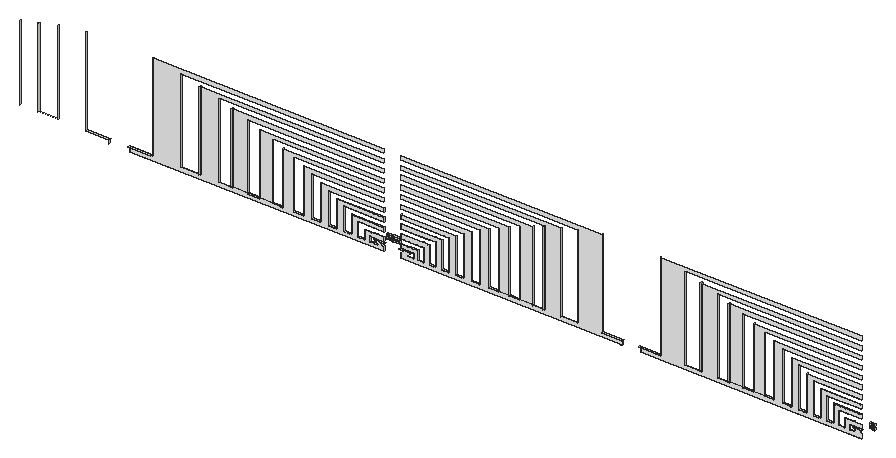
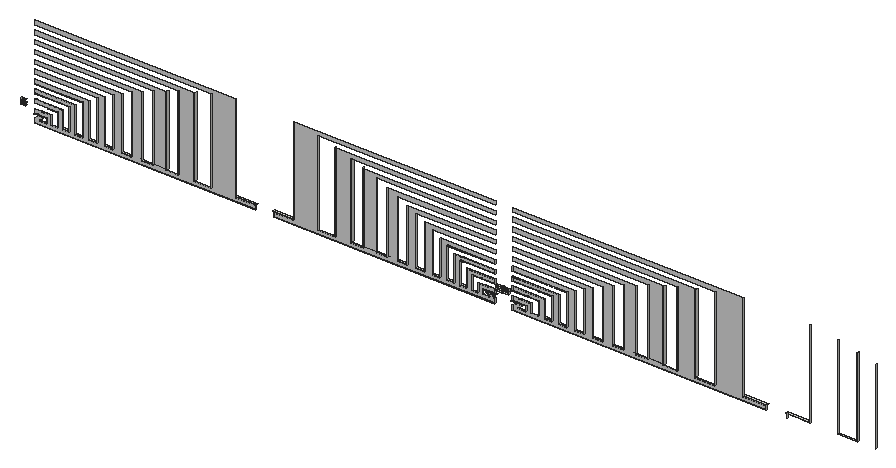
# SketchUp Ruby script. Lengths in inches.
U = 1.inch
M = Sketchup.active_model
def pt(a) = Geom::Point3d.new(a.map { |v| v * U })
def face(e, loops, mat)
  f = e.add_face(loops[0].map { |a| pt(a) })
  loops[1..].each { |l| e.add_face(l.map { |a| pt(a) }).erase! }
  f.material = f.back_material = mat if mat
  f
end
# faces: each face lists its corners as indices into pts; further lists are holes
def faces(e, pts, list, mat = nil) = list.each { |f| face(e, (f[0].is_a?(Array) ? f : [f]).map { |l| l.map { |i| pts[i] } }, mat) }
# xy, xz, yz: faces in a plane at the given z, y or x. An outline is a flat list of corners, or four numbers for a rectangle; further outlines are holes
def ring(l) = l.size == 4 ? [[l[0], l[1]], [l[2], l[1]], [l[2], l[3]], [l[0], l[3]]] : l.each_slice(2).to_a
def flat(e, list, mat, &to3) = list.each { |f| face(e, (f[0].is_a?(Array) ? f : [f]).map { |l| ring(l).map { |u, v| to3.(u, v) } }, mat) }
def xy(e, z, list, mat = nil) = flat(e, list, mat) { |x, y| [x, y, z] }
def xz(e, y, list, mat = nil) = flat(e, list, mat) { |x, z| [x, y, z] }
def yz(e, x, list, mat = nil) = flat(e, list, mat) { |y, z| [x, y, z] }
def lines(e, pts, list) = list.each { |a, b| e.add_line(pt(pts[a]), pt(pts[b])) }
# prism: a flat outline (further loops are holes) pulled along v
def prism(e, loops, v, mat = nil)
  f = face(e, loops, mat); d = Geom::Vector3d.new(v.map { |x| x * U })
  f.pushpull(f.normal.samedirection?(d) ? d.length : -d.length)
end
def box(e, o, s, mat = nil) = prism(e, [[o, [o[0] + s[0], o[1], o[2]], [o[0] + s[0], o[1] + s[1], o[2]], [o[0], o[1] + s[1], o[2]]]], [0, 0, s[2]], mat)
def at(x, y, z, deg = 0) = Geom::Transformation.translation(pt([x, y, z])) * Geom::Transformation.rotation(ORIGIN, Z_AXIS, deg.degrees)
def axes(o, x, y, z) = Geom::Transformation.new([*x, 0, *y, 0, *z, 0, *pt(o).to_a, 1])
def part(name) = M.definitions.add(name)
# library, detail: a bought-in or finely detailed component or shape, given as its bounding box
def library(name, o, s) = part(name).tap { |d| box(d.entities, o, s) }
def detail(e, o, s) = box(e.add_group.entities, o, s)
def put(e, d, t, mat = nil) = e.add_instance(d, t).tap { |i| i.material = mat if mat }
def group(e, t, mat = nil) = e.add_group.tap { |g| g.transformation = t; g.material = mat if mat }.entities
root = M.entities
M.materials.add("[Color_000]").color = [255, 255, 255]
xy(root,0.49,[[835.26,13.81,1012.48,14.31],[1024.39,13.81,1178.58,14.31],[1191.27,13.81,1345.46,14.31]])
xy(root,3.2,[[771.16,13.81,785.19,14.31],[804.64,13.81,816.11,14.31],[816.11,13.81,820.67,14.31],[835.26,13.81,839.82,14.31],[839.82,13.81,851.28,14.31],
  [870.74,13.81,884.76,14.31],[897.07,13.81,907.12,14.31],[917.52,13.81,926.1,14.31],[934.55,13.81,942.21,14.31],[949.3125,13.81,956.23,14.31],
  [962.35,13.81,968.64,14.31],[974.05,13.81,979.79,14.31],[984.5625,13.81,989.91,14.31],[993.96,13.81,999.18,14.31],[1002.58,13.81,1008.33,14.31],
  [1028,13.81,1033,14.31],[1035.96,13.81,1040.51,14.31],[1044.03,13.81,1048.68,14.31],[1052.83,13.81,1057.83,14.31],[1062.53,13.81,1068,14.31],
  [1073.33,13.81,1079.35,14.31],[1085.53,13.81,1092.19,14.31],[1099.55,13.81,1107,14.31],[1116.06,13.81,1124.8,14.31],[1135.51,13.81,1147.71,14.31],
  [1164.63,13.81,1174.61,14.31],[1174.61,13.81,1178.58,14.31],[1191.27,13.81,1195.24,14.31],[1195.24,13.81,1205.21,14.31],[1222.14,13.81,1234.34,14.31],
  [1245.05,13.81,1253.79,14.31],[1262.84,13.81,1270.3,14.31],[1277.65,13.81,1284.32,14.31],[1290.5,13.81,1296.52,14.31],[1301.84,13.81,1307.3125,14.31],
  [1312.02,13.81,1317.01,14.31],[1321.17,13.81,1325.82,14.31],[1329.34,13.81,1333.88,14.31],[1336.84,13.81,1341.84,14.31]])
xy(root,3.7,[[805.43,12.93,821.45,14.31],[834.47,12.93,850.5,14.31],[1165.32,12.93,1179.26,14.31],[1190.59,12.93,1204.53,14.31],[989.12,13.04,985.35,13.08,985.35,14.31,989.12,14.31],
  [1044.71,13.04,1047.99,13.08,1047.99,14.31,1044.71,14.31],[1325.13,13.04,1321.85,13.08,1321.85,14.31,1325.13,14.31],[979,13.15,974.83,13.19,974.83,14.31,979,14.31],[1053.52,13.15,1057.15,13.19,1057.15,14.31,1053.52,14.31],[1316.33,13.15,1312.7,13.19,1312.7,14.31,1316.33,14.31],
  [967.85,13.27,963.14,13.32,963.14,14.31,967.85,14.31],[1063.22,13.27,1067.32,13.32,1067.32,14.31,1063.22,14.31],[1306.63,13.27,1302.53,13.32,1302.53,14.31,1306.63,14.31],[955.44,13.4,950.1,13.46,950.1,14.31,955.44,14.31],[1074.02,13.4,1078.67,13.46,1078.67,14.31,1074.02,14.31],
  [1295.83,13.4,1291.18,13.46,1291.18,14.31,1295.83,14.31],[941.43,13.55,935.33,13.62,935.33,14.31,941.43,14.31],[1086.21,13.55,1091.51,13.62,1091.51,14.31,1086.21,14.31],[1283.64,13.55,1278.34,13.62,1278.34,14.31,1283.64,14.31],[925.31,13.73,918.3125,13.8,918.3125,14.31,925.31,14.31],
  [1100.23,13.73,1106.32,13.8,1106.32,14.31,1100.23,14.31],[1269.61,13.73,1263.53,13.8,1263.53,14.31,1269.61,14.31]])
xy(root,5.63,[[1005.07,13.81,1009.64,14.31],[1026.86,13.81,1030.84,14.31]])
xy(root,6.12,[[1010.01,12.93,1013.27,14.31],[1023.71,12.93,1026.55,14.31],[1343.3,12.93,1346.14,14.31]])
xy(root,6.62,[[1002.58,13.81,1010.01,14.31],[1010.01,13.81,1011.13,14.31],[1011.13,13.81,1012.48,14.31],[1024.39,13.81,1025.57,14.31],[1025.57,13.81,1026.55,14.31],
  [1026.55,13.81,1033,14.31],[1336.84,13.81,1343.3,14.31]])
xy(root,9.21,[[1014.6875,13.24,1018.58,14.43],[1019.16,13.24,1023.63,14.43],[1351.27,13.24,1355.16,14.43]])
xy(root,9.32,[[999.18,13.81,1005.03,14.31],[1005.03,13.81,1006.64,14.31],[1006.64,13.81,1012.48,14.31],[1024.39,13.81,1029.48,14.31],[1029.48,13.81,1030.875,14.31],
  [1030.875,13.81,1035.96,14.31],[1333.88,13.81,1338.97,14.31],[1338.97,13.81,1340.37,14.31]])
xy(root,10.5,[[1014.6875,13.24,1018.58,14.43],[1019.16,13.24,1023.63,14.43],[1351.27,13.24,1355.16,14.43]])
xy(root,11.42,[[1014.6875,13.24,1018.58,14.43],[1019.16,13.24,1023.63,14.43],[1351.27,13.24,1355.16,14.43]])
xy(root,12.71,[[1014.6875,13.24,1018.58,14.43],[1019.16,13.24,1023.63,14.43],[1351.27,13.24,1355.16,14.43]])
xy(root,12.74,[[993.96,13.81,1001.75,14.31],[1001.75,13.81,1012.48,14.31],[1024.39,13.81,1033.73,14.31],[1033.73,13.81,1040.51,14.31],[1329.34,13.81,1336.12,14.31]])
xy(root,15.44,[[989.91,13.81,996.13,14.31],[996.13,13.81,1012.48,14.31],[1024.39,13.81,1038.62,14.31],[1038.62,13.81,1044.03,14.31],[1325.82,13.81,1331.23,14.31],
  [1331.23,13.81,1345.46,14.31]])
xy(root,18.86,[[984.5625,13.81,992.44,14.31],[992.44,13.81,1012.48,14.31],[1024.39,13.81,1041.83,14.31],[1041.83,13.81,1048.68,14.31],[1321.17,13.81,1328.02,14.31],
  [1328.02,13.81,1345.46,14.31]])
xy(root,21.57,[[979.79,13.81,986.45,14.31],[986.45,13.81,1012.48,14.31],[1024.39,13.81,1047.04,14.31],[1047.04,13.81,1052.83,14.31],[1317.01,13.81,1322.8125,14.31],
  [1322.8125,13.81,1345.46,14.31]])
xy(root,24.98,[[974.05,13.81,982.29,14.31],[982.29,13.81,1012.48,14.31],[1024.39,13.81,1050.66,14.31],[1050.66,13.81,1057.83,14.31],[1312.02,13.81,1319.1875,14.31],
  [1319.1875,13.81,1345.46,14.31]])
xz(root,13.81,[[835.26,0.49,1012.48,0.49,1012.48,3.52,1009.64,5.63,1005.07,5.63,1008.33,3.2,1002.58,3.2,1002.58,6.62,1012.48,6.62,1012.48,9.32,999.18,9.32,999.18,3.2,993.96,3.2,993.96,12.74,1012.48,12.74,1012.48,15.44,989.91,15.44,989.91,3.2,984.5625,3.2,984.5625,18.86,1012.48,18.86,1012.48,21.57,979.79,21.57,979.79,3.2,974.05,3.2,974.05,24.98,1012.48,24.98,1012.48,27.6875,968.64,27.6875,968.64,3.2,962.35,3.2,962.35,31.1,1012.48,31.1,1012.48,33.81,956.23,33.81,956.23,3.2,949.3125,3.2,949.3125,37.22,1012.48,37.22,1012.48,39.93,942.21,39.93,942.21,3.2,934.55,3.2,934.55,43.34,1012.48,43.34,1012.48,46.05,926.1,46.05,926.1,3.2,917.52,3.2,917.52,49.46,1012.48,49.46,1012.48,52.17,907.12,52.17,907.12,3.2,897.07,3.2,897.07,55.59,1012.48,55.59,1012.48,58.29,884.76,58.29,884.76,3.2,870.74,3.2,870.74,61.71,1012.48,61.71,1012.48,64.41,851.28,64.41,851.28,3.2,835.26,3.2],[1024.39,0.49,1024.39,3.52,1026.86,5.63,1030.84,5.63,1028,3.2,1033,3.2,1033,6.62,1024.39,6.62,1024.39,9.32,1035.96,9.32,1035.96,3.2,1040.51,3.2,1040.51,12.74,1024.39,12.74,1024.39,15.44,1044.03,15.44,1044.03,3.2,1048.68,3.2,1048.68,18.86,1024.39,18.86,1024.39,21.57,1052.83,21.57,1052.83,3.2,1057.83,3.2,1057.83,24.98,1024.39,24.98,1024.39,27.6875,1062.53,27.6875,1062.53,3.2,1068,3.2,1068,31.1,1024.39,31.1,1024.39,33.81,1073.33,33.81,1073.33,3.2,1079.35,3.2,1079.35,37.22,1024.39,37.22,1024.39,39.93,1085.53,39.93,1085.53,3.2,1092.19,3.2,1092.19,43.34,1024.39,43.34,1024.39,46.05,1099.55,46.05,1099.55,3.2,1107,3.2,1107,49.46,1024.39,49.46,1024.39,52.17,1116.06,52.17,1116.06,3.2,1124.8,3.2,1124.8,55.59,1024.39,55.59,1024.39,58.29,1135.51,58.29,1135.51,3.2,1147.71,3.2,1147.71,61.71,1024.39,61.71,1024.39,64.41,1164.63,64.41,1164.63,3.2,1178.58,3.2,1178.58,0.49],[1191.27,0.49,1345.46,0.49,1345.46,3.52,1342.98,5.63,1339,5.63,1341.84,3.2,1336.84,3.2,1336.84,6.62,1345.46,6.62,1345.46,9.32,1333.88,9.32,1333.88,3.2,1329.34,3.2,1329.34,12.74,1345.46,12.74,1345.46,15.44,1325.82,15.44,1325.82,3.2,1321.17,3.2,1321.17,18.86,1345.46,18.86,1345.46,21.57,1317.01,21.57,1317.01,3.2,1312.02,3.2,1312.02,24.98,1345.46,24.98,1345.46,27.6875,1307.3125,27.6875,1307.3125,3.2,1301.84,3.2,1301.84,31.1,1345.46,31.1,1345.46,33.81,1296.52,33.81,1296.52,3.2,1290.5,3.2,1290.5,37.22,1345.46,37.22,1345.46,39.93,1284.32,39.93,1284.32,3.2,1277.65,3.2,1277.65,43.34,1345.46,43.34,1345.46,46.05,1270.3,46.05,1270.3,3.2,1262.84,3.2,1262.84,49.46,1345.46,49.46,1345.46,52.17,1253.79,52.17,1253.79,3.2,1245.05,3.2,1245.05,55.59,1345.46,55.59,1345.46,58.29,1234.34,58.29,1234.34,3.2,1222.14,3.2,1222.14,61.71,1345.46,61.71,1345.46,64.41,1205.21,64.41,1205.21,3.2,1191.27,3.2]],"[Color_000]")
yz(root,758.85,[[13.81,3.2,14.31,55.59]])
yz(root,771.16,[[13.81,3.2,14.31,58.29]])
yz(root,771.95,[[12.93,3.7,14.31,58.6]])
yz(root,785.19,[[13.81,3.2,14.31,61.71]])
yz(root,804.64,[[13.81,3.2,14.31,64.41]])
yz(root,820.67,[[13.81,0.49,14.31,3.2]])
yz(root,835.26,[[13.81,0.49,14.31,3.2]])
yz(root,851.28,[[13.81,3.2,14.31,64.41]])
yz(root,870.74,[[13.81,3.2,14.31,61.71]])
yz(root,883.97,[[12.93,3.7,14.31,58.6]])
yz(root,884.76,[[13.81,3.2,14.31,58.29]])
yz(root,897.07,[[13.81,3.2,14.31,55.59]])
yz(root,897.86,[[12.93,3.7,14.31,55.09]])
yz(root,906.33,[[12.93,3.7,14.31,52.67]])
yz(root,907.12,[[13.81,3.2,14.31,52.17]])
yz(root,917.52,[[13.81,3.2,14.31,49.46]])
yz(root,926.1,[[13.81,3.2,14.31,46.05]])
yz(root,934.55,[[13.81,3.2,14.31,43.34]])
yz(root,942.21,[[13.81,3.2,14.31,39.93]])
yz(root,949.3125,[[13.81,3.2,14.31,37.22]])
yz(root,956.23,[[13.81,3.2,14.31,33.81]])
yz(root,962.35,[[13.81,3.2,14.31,31.1]])
yz(root,968.64,[[13.81,3.2,14.31,27.6875]])
yz(root,974.05,[[13.81,3.2,14.31,24.98]])
yz(root,979.79,[[13.81,3.2,14.31,21.57]])
yz(root,984.5625,[[13.81,3.2,14.31,18.86]])
yz(root,989.91,[[13.81,3.2,14.31,15.44]])
yz(root,993.96,[[13.81,3.2,14.31,12.74]])
yz(root,999.18,[[13.81,3.2,14.31,9.32]])
yz(root,1002.58,[[13.81,3.2,14.31,6.62]])
yz(root,1012.48,[[13.81,0.49,14.31,3.52],[13.81,6.62,14.31,9.32],[13.81,12.74,14.31,15.44],[13.81,18.86,14.31,21.57],[13.81,24.98,14.31,27.6875]])
yz(root,1014.6875,[[13.24,9.21,14.43,10.5],[13.24,11.42,14.43,12.71]])
yz(root,1023.63,[[13.24,9.21,14.43,10.5],[13.24,11.42,14.43,12.71]])
yz(root,1024.39,[[13.81,0.49,14.31,3.52],[13.81,6.62,14.31,9.32],[13.81,12.74,14.31,15.44],[13.81,18.86,14.31,21.57],[13.81,24.98,14.31,27.6875]])
yz(root,1033,[[13.81,3.2,14.31,6.62]])
yz(root,1035.96,[[13.81,3.2,14.31,9.32]])
yz(root,1040.51,[[13.81,3.2,14.31,12.74]])
yz(root,1044.03,[[13.81,3.2,14.31,15.44]])
yz(root,1048.68,[[13.81,3.2,14.31,18.86]])
yz(root,1052.83,[[13.81,3.2,14.31,21.57]])
yz(root,1057.83,[[13.81,3.2,14.31,24.98]])
yz(root,1062.53,[[13.81,3.2,14.31,27.6875]])
yz(root,1068,[[13.81,3.2,14.31,31.1]])
yz(root,1073.33,[[13.81,3.2,14.31,33.81]])
yz(root,1079.35,[[13.81,3.2,14.31,37.22]])
yz(root,1085.53,[[13.81,3.2,14.31,39.93]])
yz(root,1092.19,[[13.81,3.2,14.31,43.34]])
yz(root,1099.55,[[13.81,3.2,14.31,46.05]])
yz(root,1107,[[13.81,3.2,14.31,49.46]])
yz(root,1116.06,[[13.81,3.2,14.31,52.17]])
yz(root,1116.74,[[12.93,3.7,14.31,52.67]])
yz(root,1124.11,[[12.93,3.7,14.31,55.09]])
yz(root,1124.8,[[13.81,3.2,14.31,55.59]])
yz(root,1135.51,[[13.81,3.2,14.31,58.29]])
yz(root,1136.19,[[12.93,3.7,14.31,58.6]])
yz(root,1147.71,[[13.81,3.2,14.31,61.71]])
yz(root,1164.63,[[13.81,3.2,14.31,64.41]])
yz(root,1178.58,[[13.81,0.49,14.31,3.2]])
yz(root,1191.27,[[13.81,0.49,14.31,3.2]])
yz(root,1205.21,[[13.81,3.2,14.31,64.41]])
yz(root,1222.14,[[13.81,3.2,14.31,61.71]])
yz(root,1233.65,[[12.93,3.7,14.31,58.6]])
yz(root,1234.34,[[13.81,3.2,14.31,58.29]])
yz(root,1245.05,[[13.81,3.2,14.31,55.59]])
yz(root,1245.73,[[12.93,3.7,14.31,55.09]])
yz(root,1253.1,[[12.93,3.7,14.31,52.67]])
yz(root,1253.79,[[13.81,3.2,14.31,52.17]])
yz(root,1262.84,[[13.81,3.2,14.31,49.46]])
yz(root,1270.3,[[13.81,3.2,14.31,46.05]])
yz(root,1277.65,[[13.81,3.2,14.31,43.34]])
yz(root,1284.32,[[13.81,3.2,14.31,39.93]])
yz(root,1290.5,[[13.81,3.2,14.31,37.22]])
yz(root,1296.52,[[13.81,3.2,14.31,33.81]])
yz(root,1301.84,[[13.81,3.2,14.31,31.1]])
yz(root,1307.3125,[[13.81,3.2,14.31,27.6875]])
yz(root,1312.02,[[13.81,3.2,14.31,24.98]])
yz(root,1317.01,[[13.81,3.2,14.31,21.57]])
yz(root,1321.17,[[13.81,3.2,14.31,18.86]])
yz(root,1325.82,[[13.81,3.2,14.31,15.44]])
yz(root,1329.34,[[13.81,3.2,14.31,12.74]])
yz(root,1333.88,[[13.81,3.2,14.31,9.32]])
yz(root,1336.84,[[13.81,3.2,14.31,6.62]])
yz(root,1355.16,[[13.24,9.21,14.43,10.5],[13.24,11.42,14.43,12.71]])
p = [[1005.07,14.31,5.63],[1008.33,14.31,3.2],[1008.33,13.81,3.2],[1005.07,13.81,5.63],[1030.84,14.31,5.63],[1028,14.31,3.2],
  [1028,13.81,3.2],[1030.84,13.81,5.63],[1339,14.31,5.63],[1341.84,14.31,3.2],[1341.84,13.81,3.2],[1339,13.81,5.63],
  [1012.48,14.31,3.52],[1009.64,14.31,5.63],[1009.64,13.81,5.63],[1012.48,13.81,3.52],[1024.39,14.31,3.52],[1026.86,14.31,5.63],
  [1026.86,13.81,5.63],[1024.39,13.81,3.52],[925.31,13.73,3.7],[935.33,13.62,3.7],[906.33,13.93,3.7],[918.3125,13.8,3.7],
  [1269.61,13.73,3.7],[1278.34,13.62,3.7],[1253.1,13.93,3.7],[1263.53,13.8,3.7],[1100.23,13.73,3.7],[1091.51,13.62,3.7],
  [1116.74,13.93,3.7],[1106.32,13.8,3.7]]
faces(root,p,[[0,1,2,3],[4,5,6,7],[8,9,10,11],[12,13,14,15],[16,17,18,19]])
lines(root,p,[[20,21],[22,23],[24,25],[26,27],[28,29],[30,31]])
